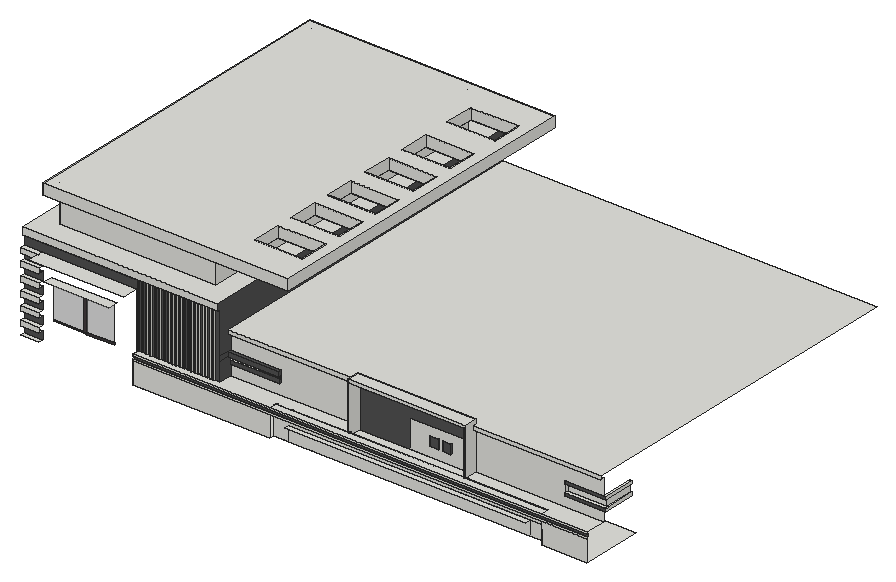
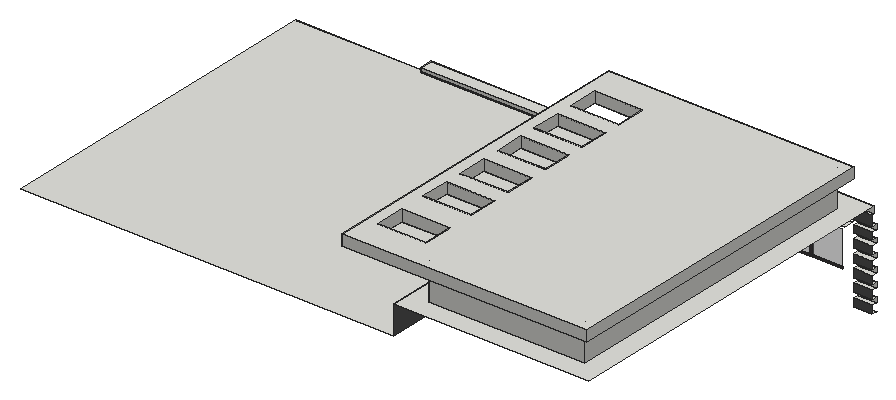
# SketchUp Ruby script. Lengths in inches.
U = 1.inch
M = Sketchup.active_model
def pt(a) = Geom::Point3d.new(a.map { |v| v * U })
def face(e, loops, mat)
  f = e.add_face(loops[0].map { |a| pt(a) })
  loops[1..].each { |l| e.add_face(l.map { |a| pt(a) }).erase! }
  f.material = f.back_material = mat if mat
  f
end
# faces: each face lists its corners as indices into pts; further lists are holes
def faces(e, pts, list, mat = nil) = list.each { |f| face(e, (f[0].is_a?(Array) ? f : [f]).map { |l| l.map { |i| pts[i] } }, mat) }
# xy, xz, yz: faces in a plane at the given z, y or x. An outline is a flat list of corners, or four numbers for a rectangle; further outlines are holes
def ring(l) = l.size == 4 ? [[l[0], l[1]], [l[2], l[1]], [l[2], l[3]], [l[0], l[3]]] : l.each_slice(2).to_a
def flat(e, list, mat, &to3) = list.each { |f| face(e, (f[0].is_a?(Array) ? f : [f]).map { |l| ring(l).map { |u, v| to3.(u, v) } }, mat) }
def xy(e, z, list, mat = nil) = flat(e, list, mat) { |x, y| [x, y, z] }
def xz(e, y, list, mat = nil) = flat(e, list, mat) { |x, z| [x, y, z] }
def yz(e, x, list, mat = nil) = flat(e, list, mat) { |y, z| [x, y, z] }
def lines(e, pts, list) = list.each { |a, b| e.add_line(pt(pts[a]), pt(pts[b])) }
# prism: a flat outline (further loops are holes) pulled along v
def prism(e, loops, v, mat = nil)
  f = face(e, loops, mat); d = Geom::Vector3d.new(v.map { |x| x * U })
  f.pushpull(f.normal.samedirection?(d) ? d.length : -d.length)
end
def box(e, o, s, mat = nil) = prism(e, [[o, [o[0] + s[0], o[1], o[2]], [o[0] + s[0], o[1] + s[1], o[2]], [o[0], o[1] + s[1], o[2]]]], [0, 0, s[2]], mat)
def at(x, y, z, deg = 0) = Geom::Transformation.translation(pt([x, y, z])) * Geom::Transformation.rotation(ORIGIN, Z_AXIS, deg.degrees)
def axes(o, x, y, z) = Geom::Transformation.new([*x, 0, *y, 0, *z, 0, *pt(o).to_a, 1])
def part(name) = M.definitions.add(name)
# library, detail: a bought-in or finely detailed component or shape, given as its bounding box
def library(name, o, s) = part(name).tap { |d| box(d.entities, o, s) }
def detail(e, o, s) = box(e.add_group.entities, o, s)
def put(e, d, t, mat = nil) = e.add_instance(d, t).tap { |i| i.material = mat if mat }
def group(e, t, mat = nil) = e.add_group.tap { |g| g.transformation = t; g.material = mat if mat }.entities
root = M.entities
M.materials.add("[0128_White]").color = [255, 255, 255]
M.materials.add("[0135_DarkGray]").color = [81, 81, 81]
M.materials.add("[Asphalt New]").color = [67, 60, 62]
M.materials.add("[Translucent Glass Gray]").color = [128, 128, 128]
M.materials["[Translucent Glass Gray]"].alpha = 0.5
xy(root,609.09,[[754.01,573.8,754.01,587.17,900.26,587.17,900.26,588.61,910.24,588.61,910.24,691.875,1630.5,691.875,1630.5,573.8,1541.95,573.8,1541.95,584.05,1018.16,584.05,1018.16,573.8]])
xy(root,610.34,[[751.95,587.17,751.95,588.61,759.72,588.61,759.72,587.25],[759.72,587.17,759.72,587.25,761.63,587.26,761.63,587.17],[826.47,587.17,826.47,587.89,828.38,587.91,828.38,587.17],[833.72,587.17,833.72,587.96,835.63,587.98,835.63,587.17],[840.97,587.17,840.97,588.03,842.88,588.05,842.88,587.17],
  [848.22,587.17,848.22,588.1,850.13,588.12,850.13,587.17],[855.47,587.17,855.47,588.17,857.38,588.19,857.38,587.17],[862.72,587.17,862.72,588.24,864.63,588.26,864.63,587.17],[864.63,587.17,864.63,588.26,900.26,588.61,900.26,587.17],[759.72,587.25,759.72,588.61,761.63,588.61,761.63,587.26],
  [761.63,587.26,761.63,588.61,826.47,588.61,826.47,587.89],[826.47,587.89,826.47,588.61,828.38,588.61,828.38,587.91],[828.38,587.91,828.38,588.61,833.72,588.61,833.72,587.96],[833.72,587.96,833.72,588.61,835.63,588.61,835.63,587.98],[835.63,587.98,840.97,588.03,840.97,588.61,835.63,588.61],
  [840.97,588.03,842.88,588.05,842.88,588.61,840.97,588.61],[842.88,588.05,848.22,588.1,850.13,588.12,855.47,588.17,855.47,588.61,842.88,588.61],[855.47,588.17,855.47,588.61,857.38,588.61,857.38,588.19],[857.38,588.19,857.38,588.61,862.72,588.61,862.72,588.24],[862.72,588.24,862.72,588.61,864.63,588.61,864.63,588.26],
  [864.63,588.26,864.63,588.61,900.26,588.61]])
xy(root,613.14,[[768.22,587.17,770.13,588.61]])
xy(root,614.21,[[833.72,587.17,835.63,588.61]])
xy(root,614.94,[[532.875,578.55,567.67,588.61]])
xy(root,617.71,[[848.22,588.1,848.22,588.61,850.13,588.61,850.13,588.12]])
xy(root,618.02,[[802.22,587.17,804.13,588.61]])
xy(root,618.27,[[776.72,587.17,778.63,588.61]])
xy(root,619.64,[[751.95,587.17,753.71,588.61]])
xy(root,619.89,[[751.95,587.17,753.71,588.61]])
xy(root,620.96,[[810.72,587.17,812.63,588.61]])
xy(root,621.14,[[785.22,587.17,787.13,588.61]])
xy(root,621.58,[[819.22,587.17,821.13,588.61]])
xy(root,622.21,[[793.72,587.17,795.63,588.61]])
xy(root,630.78,[[532.875,578.55,567.67,588.61]])
xy(root,637.28,[[1047.4,573.8,1512.22,584.05]])
xy(root,640.5,[[532.875,578.55,567.67,588.61]])
xy(root,653.49,[[754.01,573.8,1630.5,576.11]])
xy(root,656.34,[[532.875,578.55,567.67,588.61]])
xy(root,656.4,[[1018.16,584.05,1541.95,588.61],[1158.77,588.61,1380.86,613.8125]])
xy(root,658.77,[[754.01,573.8,1630.5,576.11]])
xy(root,662.4375,[[1018.14,588.61,1047.4,628.55]])
xy(root,662.46,[[754.01,573.8,1018.16,573.8,1018.16,588.61,1155.85,588.61,1155.85,613.8125,910.24,613.8125,910.24,588.61,900.26,588.61,900.26,587.17,754.01,587.17],[1018.16,573.8,1541.95,588.61],[1541.95,573.8,1630.5,573.8,1630.5,613.8125,1383.78,613.8125,1383.78,588.61,1541.95,588.61]])
xy(root,666.07,[[532.875,578.55,567.67,588.61]])
xy(root,676.27,[[1295.68,612.0625,1312.87,613.8125],[1320.3,612.0625,1337.49,613.8125]])
xy(root,681.07,[[1556.35,612.75,1633.375,613.8125],[1633.375,612.75,1633.375,613.8125,1630.5,613.8125,1630.5,676.48,1634.625,676.48,1634.625,612.75]])
xy(root,681.9,[[532.875,578.55,567.67,588.61]])
xy(root,683.37,[[910.24,611.625,1007.99,613.8125]],"[0135_DarkGray]")
xy(root,687.32,[[1556.35,612.75,1633.375,612.75,1633.375,617.9375,1629.9375,617.9375,1629.9375,620.0625,1556.35,620.0625],[1633.375,612.75,1634.625,612.75,1634.625,676.48,1630.5,676.48,1630.5,620.0625,1629.9375,620.0625,1629.9375,617.9375,1633.375,617.9375]])
xy(root,690.93,[[910.24,611.625,1007.99,617.5]])
xy(root,691.63,[[532.875,578.55,567.67,588.61]])
xy(root,693.46,[[1295.68,612.0625,1312.87,613.8125],[1320.3,612.0625,1337.49,613.8125]],"[0135_DarkGray]")
xy(root,697.59,[[910.24,606.92,1007.99,617.5]])
xy(root,701.62,[[1556.35,612.75,1556.35,620.0625,1629.9375,620.0625,1629.9375,617.9375,1633.375,617.9375,1633.375,613.8125,1634.8125,613.8125,1634.8125,612.75],[1633.375,613.8125,1633.375,617.9375,1629.9375,617.9375,1629.9375,620.0625,1630.5,620.0625,1630.5,676.48,1634.8125,676.48,1634.8125,613.8125]],"[0135_DarkGray]")
xy(root,706.43,[[910.24,606.92,1007.99,613.8125]],"[0135_DarkGray]")
xy(root,706.75,[[1556.35,612.75,1634.8125,613.8125],[1630.5,613.8125,1634.8125,676.48]])
xy(root,707.46,[[532.875,578.55,567.67,588.61]])
xy(root,717.19,[[532.875,578.55,567.67,588.61]])
xy(root,733.03,[[532.875,578.55,567.67,588.61]])
xy(root,737.63,[[1383.78,606.125,1630.5,613.8125],[910.24,606.625,1155.85,613.8125]])
xy(root,737.97,[[595.83,556.73,721.27,575.61]])
xy(root,742.75,[[532.875,578.55,567.67,588.61]])
xy(root,745.125,[[1383.78,606.125,1630.5,606.125,1630.5,1270.99,910.24,1270.99,910.24,606.625,1155.85,606.625,1155.85,613.8125,1383.78,613.8125],[1158.77,606.125,1380.86,613.8125]])
xy(root,747.65,[[1158.77,588.61,1380.86,613.8125]])
xy(root,753.0625,[[1155.85,588.61,1383.78,613.8125]])
xy(root,756.4,[[532.875,578.55,567.67,588.61]])
xy(root,766.13,[[567.67,556.73,749.43,588.61],[532.875,578.55,567.67,588.61]])
xy(root,786.75,[[532.875,583.8,750.55,588.61],[750.55,583.8,751.95,588.61],[751.95,583.8,753.71,587.17],[753.71,583.8,759.72,588.61],[759.72,583.8,761.63,587.17],
  [761.63,583.8,768.22,588.61],[768.22,583.8,770.13,587.17],[770.13,583.8,776.72,588.61],[776.72,583.8,778.63,587.17],[778.63,583.8,785.22,588.61],
  [785.22,583.8,787.13,587.17],[787.13,583.8,793.72,588.61],[793.72,583.8,795.63,587.17],[795.63,583.8,802.22,588.61],[802.22,583.8,804.13,587.17],
  [804.13,583.8,810.72,588.61],[810.72,583.8,812.63,587.17],[812.63,583.8,819.22,588.61],[819.22,583.8,821.13,587.17],[821.13,583.8,826.47,588.61],
  [826.47,583.8,828.38,587.17],[828.38,583.8,833.72,588.61],[833.72,583.8,835.63,587.17],[835.63,583.8,840.97,588.61],[840.97,583.8,842.88,587.17],
  [842.88,583.8,848.22,588.61],[848.22,583.8,850.13,587.17],[850.13,583.8,855.47,588.61],[855.47,583.8,857.38,587.17],[857.38,583.8,862.72,588.61],
  [862.72,583.8,864.63,587.17],[864.63,583.8,869.97,588.61],[869.97,583.8,871.88,587.17],[871.88,583.8,877.22,588.61],[877.22,583.8,879.13,587.17],
  [879.13,583.8,884.47,588.61],[884.47,583.8,886.38,587.17],[886.38,583.8,891.72,588.61],[891.72,583.8,893.63,587.17],[893.63,583.8,898.35,588.61],
  [898.35,583.8,900.26,587.17],[900.26,583.8,910.19,588.61],[910.19,583.8,910.24,588.61]])
xy(root,799.9375,[[[532.875,583.8,910.24,1270.99],[570.6,626.34,872.51,1233.27]]])
xy(root,850.625,[[[552.77,608.5,1025.6,1251.1],[570.6,626.34,872.51,1233.27],[910.47,671.07,1002.8,728.13],[910.47,759.82,1002.8,816.88],[910.47,847.45,1002.8,904.51],[910.47,937.95,1002.8,995.01],[910.47,1027.26,1002.8,1084.32],[910.47,1136.01,1002.8,1193.07]]])
xy(root,871.4375,[[[552.77,608.5,1025.6,1251.1],[910.47,671.07,1002.8,728.13],[910.47,759.82,1002.8,816.88],[910.47,847.45,1002.8,904.51],[910.47,937.95,1002.8,995.01],[910.47,1027.26,1002.8,1084.32],[910.47,1136.01,1002.8,1193.07]]])
xz(root,573.8,[[754.01,609.09,1018.16,649.875],[1541.95,609.09,1630.5,649.875],[754.01,649.875,1630.5,653.49],[754.01,658.77,1630.5,662.46]])
xz(root,575.61,[[600.1,663.68,658.55,666.89],[658.55,663.68,664.15,666.89],[664.15,663.68,716.99,666.89],[658.55,666.89,664.15,733.69]],"[Asphalt New]")
xz(root,575.61,[[600.1,666.89,658.55,733.69],[664.15,666.89,716.99,733.69]],"[Translucent Glass Gray]")
xz(root,576.11,[[754.01,653.49,1630.5,658.77]],"[0135_DarkGray]")
xz(root,578.55,[[532.875,630.78,567.67,640.5],[532.875,656.34,567.67,666.07],[532.875,681.9,567.67,691.63],[532.875,707.46,567.67,717.19],[532.875,733.03,567.67,742.75],
  [532.875,756.4,567.67,766.13]])
xz(root,583.8,[[532.875,786.75,910.24,799.9375]])
xz(root,584.05,[[1018.16,609.09,1047.4,609.09,1047.4,637.28,1541.95,637.28,1541.95,656.4,1018.16,656.4],[1047.4,609.09,1512.22,637.28],[1512.22,609.09,1541.95,637.28]])
xz(root,587.17,[[754.01,609.09,759.72,662.46],[759.72,609.09,761.63,610.34],[761.63,609.09,768.22,662.46],[768.22,609.09,770.13,613.14],[770.13,609.09,776.72,662.46],
  [776.72,609.09,778.63,618.27],[778.63,609.09,785.22,662.46],[785.22,609.09,787.13,621.14],[787.13,609.09,793.72,662.46],[793.72,609.09,795.63,622.21],
  [795.63,609.09,802.22,662.46],[802.22,609.09,804.13,618.02],[804.13,609.09,810.72,662.46],[810.72,609.09,812.63,620.96],[812.63,609.09,819.22,662.46],
  [819.22,609.09,821.13,621.58],[821.13,609.09,826.47,662.46],[826.47,609.09,828.38,610.34],[828.38,609.09,833.72,662.46],[833.72,609.09,835.63,610.34],
  [835.63,609.09,840.97,662.46],[840.97,609.09,842.88,610.34],[842.88,609.09,848.22,662.46],[848.22,609.09,850.13,610.34],[850.13,609.09,855.47,662.46],
  [855.47,609.09,857.38,610.34],[857.38,609.09,862.72,662.46],[862.72,609.09,864.63,610.34],[864.63,609.09,869.97,610.34],[869.97,609.09,871.88,610.34],
  [871.88,609.09,877.22,610.34],[877.22,609.09,879.13,610.34],[879.13,609.09,884.47,610.34],[884.47,609.09,886.38,610.34],[886.38,609.09,891.72,610.34],
  [891.72,609.09,893.63,610.34],[893.63,609.09,898.35,610.34],[898.35,609.09,900.26,610.34],[753.71,610.29,753.71,619.64,751.95,619.64,751.95,610.34],[759.72,610.34,761.63,662.46],
  [826.47,610.34,828.38,662.46],[833.72,610.34,835.63,614.21],[840.97,610.34,842.88,662.46],[848.22,610.34,850.13,662.46],[855.47,610.34,857.38,662.46],
  [862.72,610.34,864.63,662.46],[864.63,610.34,869.97,662.46],[869.97,610.34,871.88,662.46],[871.88,610.34,877.22,662.46],[877.22,610.34,879.13,662.46],
  [879.13,610.34,884.47,662.46],[884.47,610.34,886.38,662.46],[886.38,610.34,891.72,662.46],[891.72,610.34,893.63,662.46],[893.63,610.34,898.35,662.46],
  [898.35,610.34,900.26,662.46],[768.22,613.14,770.13,662.46],[833.72,614.21,835.63,662.46],[802.22,618.02,804.13,662.46],[776.72,618.27,778.63,662.46],
  [751.95,619.64,753.71,619.89],[751.95,619.89,753.71,786.75],[810.72,620.96,812.63,662.46],[785.22,621.14,787.13,662.46],[819.22,621.58,821.13,662.46],
  [793.72,622.21,795.63,662.46],[759.72,662.46,761.63,786.75],[768.22,662.46,770.13,786.75],[776.72,662.46,778.63,786.75],[785.22,662.46,787.13,786.75],
  [793.72,662.46,795.63,786.75],[802.22,662.46,804.13,786.75],[810.72,662.46,812.63,786.75],[819.22,662.46,821.13,786.75],[826.47,662.46,828.38,786.75],
  [833.72,662.46,835.63,786.75],[840.97,662.46,842.88,786.75],[869.97,662.46,871.88,786.75],[877.22,662.46,879.13,786.75],[884.47,662.46,886.38,786.75],
  [891.72,662.46,893.63,786.75],[898.35,662.46,900.26,786.75]])
xz(root,587.17,[[848.22,662.46,850.13,786.75],[855.47,662.46,857.38,786.75],[862.72,662.46,864.63,786.75]],"[0128_White]")
xz(root,588.61,[[753.71,610.29,751.95,610.34,753.71,610.34],[751.95,610.34,753.71,619.64],[833.72,610.34,835.63,614.21],[751.95,619.64,753.71,619.89],[1018.16,656.4,1047.4,662.4375],
  [1047.4,656.4,1155.85,662.4375],[1155.85,656.4,1158.77,662.4375],[1158.77,656.4,1380.86,662.4375],[1380.86,656.4,1383.78,662.4375],[1383.78,656.4,1541.95,662.4375],
  [1018.16,662.4375,1047.4,662.46],[1047.4,662.4375,1155.85,662.46],[1155.85,662.4375,1158.77,662.46],[1158.77,662.4375,1380.86,662.46],[1380.86,662.4375,1383.78,662.46],
  [1383.78,662.4375,1541.95,662.46],[910.19,662.46,910.24,786.75],[1155.85,662.46,1158.77,662.46,1158.77,747.65,1380.86,747.65,1380.86,662.46,1383.78,662.46,1383.78,753.0625,1155.85,753.0625]])
xz(root,588.61,[[749.43,610.34,751.95,610.34,751.95,786.75,532.875,786.75,532.875,766.13,749.43,766.13],[753.71,610.34,759.72,786.75],[761.63,610.34,826.47,610.34,826.47,786.75,821.13,786.75,821.13,621.58,819.22,621.58,819.22,786.75,812.63,786.75,812.63,620.96,810.72,620.96,810.72,786.75,804.13,786.75,804.13,618.02,802.22,618.02,802.22,786.75,795.63,786.75,795.63,622.21,793.72,622.21,793.72,786.75,787.13,786.75,787.13,621.14,785.22,621.14,785.22,786.75,778.63,786.75,778.63,618.27,776.72,618.27,776.72,786.75,770.13,786.75,770.13,613.14,768.22,613.14,768.22,786.75,761.63,786.75],[828.38,610.34,833.72,786.75],[835.63,610.34,840.97,786.75],
  [842.88,610.34,855.47,610.34,855.47,786.75,850.13,786.75,850.13,617.71,848.22,617.71,848.22,786.75,842.88,786.75],[857.38,610.34,862.72,786.75],[864.63,610.34,869.97,786.75],[871.88,610.34,877.22,786.75],[879.13,610.34,884.47,786.75],
  [886.38,610.34,891.72,786.75],[893.63,610.34,898.35,786.75],[532.875,614.94,567.67,630.78],[532.875,640.5,567.67,656.34],[900.26,662.46,910.19,786.75],
  [532.875,666.07,567.67,681.9],[532.875,691.63,567.67,707.46],[532.875,717.19,567.67,733.03],[532.875,742.75,567.67,756.4]],"[0135_DarkGray]")
xz(root,606.125,[[1158.77,735.22,1380.86,737.6,1380.86,745.125,1158.77,745.125],[1383.78,737.63,1630.5,745.125]])
xz(root,606.625,[[910.24,737.63,1155.85,745.125]])
xz(root,606.92,[[910.24,697.59,1007.99,706.43]],"[0135_DarkGray]")
xz(root,608.5,[[552.77,850.625,1025.6,871.4375]])
xz(root,611.625,[[910.24,683.37,1007.99,690.93]],"[0135_DarkGray]")
xz(root,612.0625,[[1295.68,676.27,1312.87,693.46],[1320.3,676.27,1337.49,693.46]],"[0135_DarkGray]")
xz(root,612.75,[[1556.35,681.07,1634.625,687.32],[1556.35,701.62,1634.8125,706.75]],"[0135_DarkGray]")
xz(root,613.8125,[[[1256.73,656.4,1380.86,711.28],[1295.68,676.27,1312.87,693.46],[1320.3,676.27,1337.49,693.46]],[910.24,662.46,1155.85,662.46,1155.85,737.63,910.24,737.63,910.24,706.43,1007.99,706.43,1007.99,683.37,910.24,683.37],[1383.78,662.46,1630.5,662.46,1630.5,681.07,1556.35,681.07,1556.35,706.75,1630.5,706.75,1630.5,737.63,1383.78,737.63],[1380.86,737.6,1383.78,737.63,1383.78,745.125,1380.86,745.125],[1155.85,745.125,1155.85,753.0625,1383.78,753.0625,1383.78,745.125,1380.86,745.125,1380.86,747.65,1158.77,747.65,1158.77,745.125],
  [1158.77,745.125,1380.86,747.65]])
xz(root,613.8125,[[1158.77,656.4,1256.73,656.4,1256.73,711.28,1380.86,711.28,1380.86,737.6,1158.77,735.22]],"[0135_DarkGray]")
xz(root,617.5,[[910.24,690.93,1007.99,697.59]])
xz(root,620.0625,[[1556.35,687.32,1630.5,701.62]])
xz(root,626.34,[[570.6,799.9375,872.51,850.625]])
xz(root,671.07,[[910.47,850.625,1002.8,871.4375]])
xz(root,676.48,[[1630.5,681.07,1634.625,687.32],[1630.5,701.62,1634.8125,706.75]])
xz(root,728.13,[[910.47,850.625,1002.8,871.4375]])
xz(root,759.82,[[910.47,850.625,1002.8,871.4375]])
xz(root,816.88,[[910.47,850.625,1002.8,871.4375]])
xz(root,847.45,[[910.47,850.625,1002.8,871.4375]])
xz(root,904.51,[[910.47,850.625,1002.8,871.4375]])
xz(root,937.95,[[910.47,850.625,1002.8,871.4375]])
xz(root,995.01,[[910.47,850.625,1002.8,871.4375]])
xz(root,1027.26,[[910.47,850.625,1002.8,871.4375]])
xz(root,1084.32,[[910.47,850.625,1002.8,871.4375]])
xz(root,1136.01,[[910.47,850.625,1002.8,871.4375]])
xz(root,1193.07,[[910.47,850.625,1002.8,871.4375]])
xz(root,1233.27,[[570.6,799.9375,872.51,850.625]])
xz(root,1251.1,[[552.77,850.625,1025.6,871.4375]])
yz(root,552.77,[[608.5,850.625,1251.1,871.4375]])
yz(root,570.6,[[626.34,799.9375,1233.27,850.625]])
yz(root,751.95,[[587.17,610.34,588.61,619.64],[587.17,619.64,588.61,619.89],[587.17,619.89,588.61,786.75]])
yz(root,753.71,[[587.17,610.29,588.61,619.64],[587.17,619.64,588.61,619.89],[587.17,619.89,588.61,786.75]])
yz(root,754.01,[[573.8,609.09,573.8,653.49,576.11,653.49,576.11,658.77,573.8,658.77,573.8,662.46,587.17,662.46,587.17,609.09]])
yz(root,759.72,[[587.17,610.34,588.61,786.75]])
yz(root,761.63,[[587.17,610.34,588.61,786.75]])
yz(root,768.22,[[587.17,613.14,588.61,786.75]])
yz(root,770.13,[[587.17,613.14,588.61,786.75]])
yz(root,776.72,[[587.17,618.27,588.61,786.75]])
yz(root,778.63,[[587.17,618.27,588.61,786.75]])
yz(root,785.22,[[587.17,621.14,588.61,786.75]])
yz(root,787.13,[[587.17,621.14,588.61,786.75]])
yz(root,793.72,[[587.17,622.21,588.61,786.75]])
yz(root,795.63,[[587.17,622.21,588.61,786.75]])
yz(root,802.22,[[587.17,618.02,588.61,786.75]])
yz(root,804.13,[[587.17,618.02,588.61,786.75]])
yz(root,810.72,[[587.17,620.96,588.61,786.75]])
yz(root,812.63,[[587.17,620.96,588.61,786.75]])
yz(root,819.22,[[587.17,621.58,588.61,786.75]])
yz(root,821.13,[[587.17,621.58,588.61,786.75]])
yz(root,826.47,[[587.17,610.34,588.61,786.75]])
yz(root,828.38,[[587.17,610.34,588.61,786.75]])
yz(root,833.72,[[587.17,610.34,588.61,614.21],[587.17,614.21,588.61,786.75]])
yz(root,835.63,[[587.17,610.34,588.61,614.21],[587.17,614.21,588.61,786.75]])
yz(root,840.97,[[587.17,610.34,588.61,786.75]])
yz(root,842.88,[[587.17,610.34,588.61,786.75]])
yz(root,848.22,[[587.17,610.34,587.17,786.75,588.61,786.75,588.61,617.71,588.1,617.71,588.1,610.34]])
yz(root,850.13,[[587.17,610.34,588.12,610.34,588.12,617.71,588.61,617.71,588.61,786.75,587.17,786.75]])
yz(root,855.47,[[587.17,610.34,588.61,786.75]])
yz(root,857.38,[[587.17,610.34,588.61,786.75]])
yz(root,862.72,[[587.17,610.34,588.61,786.75]])
yz(root,864.63,[[587.17,610.34,588.61,786.75]])
yz(root,872.51,[[626.34,799.9375,1233.27,850.625]])
yz(root,900.26,[[587.17,609.09,588.61,610.34],[587.17,610.34,588.61,662.46],[587.17,662.46,588.61,786.75]])
yz(root,910.24,[[588.61,662.46,613.8125,662.46,613.8125,683.37,611.625,683.37,611.625,690.93,617.5,690.93,617.5,697.59,588.61,697.59],[588.61,697.59,606.92,706.43],[588.61,706.43,613.8125,706.43,613.8125,737.63,606.625,737.63,606.625,745.125,1270.99,745.125,1270.99,799.9375,583.8,799.9375,583.8,786.75,588.61,786.75]],"[0135_DarkGray]")
yz(root,910.47,[[671.07,850.625,728.13,871.4375],[759.82,850.625,816.88,871.4375],[847.45,850.625,904.51,871.4375],[937.95,850.625,995.01,871.4375],[1027.26,850.625,1084.32,871.4375],
  [1136.01,850.625,1193.07,871.4375]])
yz(root,1002.8,[[671.07,850.625,728.13,871.4375],[759.82,850.625,816.88,871.4375],[847.45,850.625,904.51,871.4375],[937.95,850.625,995.01,871.4375],[1027.26,850.625,1084.32,871.4375],
  [1136.01,850.625,1193.07,871.4375]])
yz(root,1007.99,[[613.8125,690.93,617.5,697.59]])
yz(root,1007.99,[[611.625,683.37,613.8125,690.93],[606.92,697.59,613.8125,706.43]],"[0135_DarkGray]")
yz(root,1018.16,[[584.05,656.4,588.61,662.46]])
yz(root,1025.6,[[608.5,850.625,1251.1,871.4375]])
yz(root,1155.85,[[588.61,662.46,588.61,753.0625,613.8125,753.0625,613.8125,745.125,606.625,745.125,606.625,737.63,613.8125,737.63,613.8125,662.46]])
yz(root,1158.77,[[588.61,656.4,613.8125,656.4,613.8125,735.22,606.125,735.22,606.125,745.125,613.8125,745.125,613.8125,747.65,588.61,747.65]])
yz(root,1295.68,[[612.0625,676.27,613.8125,693.46]],"[0135_DarkGray]")
yz(root,1312.87,[[612.0625,676.27,613.8125,693.46]],"[0135_DarkGray]")
yz(root,1320.3,[[612.0625,676.27,613.8125,693.46]],"[0135_DarkGray]")
yz(root,1337.49,[[612.0625,676.27,613.8125,693.46]],"[0135_DarkGray]")
yz(root,1380.86,[[588.61,656.4,588.61,747.65,613.8125,747.65,613.8125,745.125,606.125,745.125,606.125,737.6,613.8125,737.6,613.8125,656.4],[606.125,737.6,613.8125,745.125]])
yz(root,1383.78,[[588.61,662.46,613.8125,662.46,613.8125,737.63,606.125,737.63,606.125,745.125,613.8125,745.125,613.8125,753.0625,588.61,753.0625],[606.125,737.63,613.8125,745.125]])
yz(root,1541.95,[[573.8,609.09,583.86,637.28],[583.86,609.09,584.05,637.28]])
yz(root,1556.35,[[612.75,681.07,613.8125,687.32],[613.8125,687.32,620.0625,701.62],[612.75,701.62,613.8125,706.75]])
yz(root,1630.5,[[620.0625,687.32,676.48,701.62]])
yz(root,1634.625,[[612.75,681.07,676.48,687.32]])
yz(root,1634.8125,[[612.75,701.62,676.48,706.75]])
p = [[753.71,587.17,610.29],[751.95,587.17,610.34],[751.95,588.61,610.34],[753.71,588.61,610.29],[850.13,588.12,610.34],[848.22,588.1,610.34],
  [848.22,588.1,617.71],[850.13,588.12,617.71],[1158.77,613.8125,735.22],[1380.86,613.8125,737.6],[1380.86,606.125,737.6],[1158.77,606.125,735.22],
  [570.6,626.34,850.625],[570.6,626.34,871.4375],[872.51,1233.27,850.625],[872.51,1233.27,871.4375],[570.6,1233.27,850.625],[570.6,1233.27,871.4375]]
faces(root,p,[[0,1,2,3],[4,5,6,7],[8,9,10,11]])
lines(root,p,[[12,13],[14,15],[16,17]])
